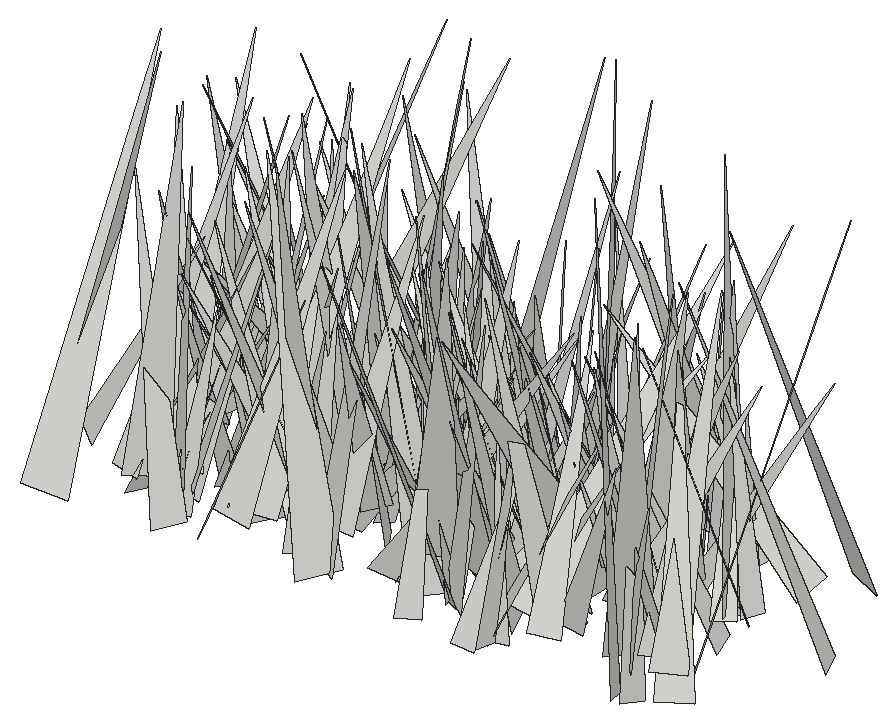
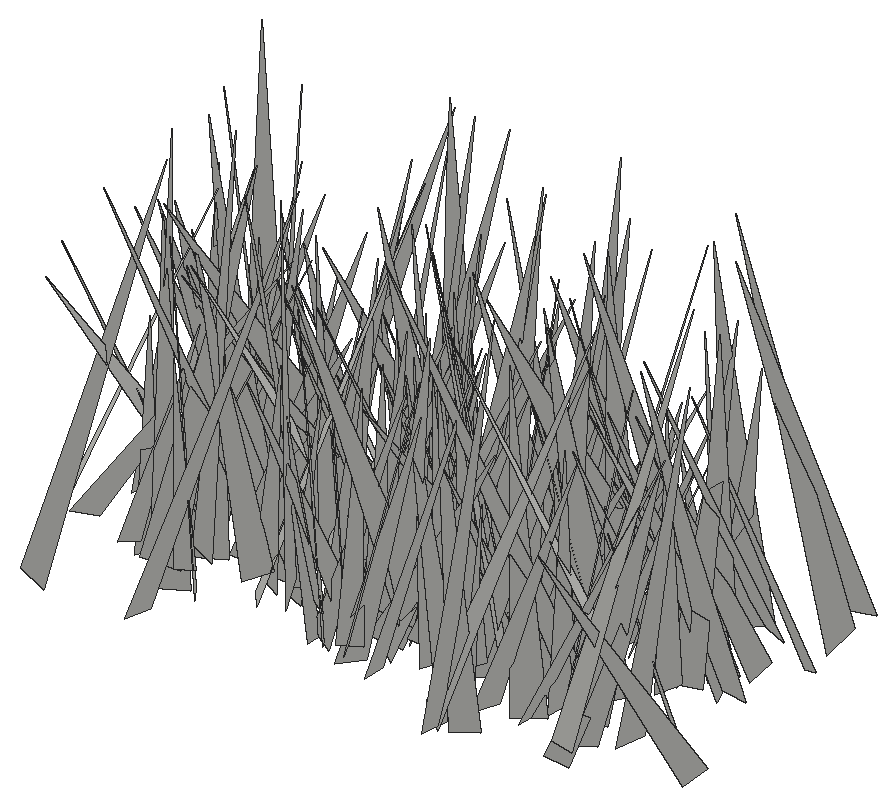
# SketchUp Ruby script. Lengths in inches.
U = 1.inch
M = Sketchup.active_model
def pt(a) = Geom::Point3d.new(a.map { |v| v * U })
def face(e, loops, mat)
  f = e.add_face(loops[0].map { |a| pt(a) })
  loops[1..].each { |l| e.add_face(l.map { |a| pt(a) }).erase! }
  f.material = f.back_material = mat if mat
  f
end
# faces: each face lists its corners as indices into pts; further lists are holes
def faces(e, pts, list, mat = nil) = list.each { |f| face(e, (f[0].is_a?(Array) ? f : [f]).map { |l| l.map { |i| pts[i] } }, mat) }
# xy, xz, yz: faces in a plane at the given z, y or x. An outline is a flat list of corners, or four numbers for a rectangle; further outlines are holes
def ring(l) = l.size == 4 ? [[l[0], l[1]], [l[2], l[1]], [l[2], l[3]], [l[0], l[3]]] : l.each_slice(2).to_a
def flat(e, list, mat, &to3) = list.each { |f| face(e, (f[0].is_a?(Array) ? f : [f]).map { |l| ring(l).map { |u, v| to3.(u, v) } }, mat) }
def xy(e, z, list, mat = nil) = flat(e, list, mat) { |x, y| [x, y, z] }
def xz(e, y, list, mat = nil) = flat(e, list, mat) { |x, z| [x, y, z] }
def yz(e, x, list, mat = nil) = flat(e, list, mat) { |y, z| [x, y, z] }
def lines(e, pts, list) = list.each { |a, b| e.add_line(pt(pts[a]), pt(pts[b])) }
# prism: a flat outline (further loops are holes) pulled along v
def prism(e, loops, v, mat = nil)
  f = face(e, loops, mat); d = Geom::Vector3d.new(v.map { |x| x * U })
  f.pushpull(f.normal.samedirection?(d) ? d.length : -d.length)
end
def box(e, o, s, mat = nil) = prism(e, [[o, [o[0] + s[0], o[1], o[2]], [o[0] + s[0], o[1] + s[1], o[2]], [o[0], o[1] + s[1], o[2]]]], [0, 0, s[2]], mat)
def at(x, y, z, deg = 0) = Geom::Transformation.translation(pt([x, y, z])) * Geom::Transformation.rotation(ORIGIN, Z_AXIS, deg.degrees)
def axes(o, x, y, z) = Geom::Transformation.new([*x, 0, *y, 0, *z, 0, *pt(o).to_a, 1])
def part(name) = M.definitions.add(name)
# library, detail: a bought-in or finely detailed component or shape, given as its bounding box
def library(name, o, s) = part(name).tap { |d| box(d.entities, o, s) }
def detail(e, o, s) = box(e.add_group.entities, o, s)
def put(e, d, t, mat = nil) = e.add_instance(d, t).tap { |i| i.material = mat if mat }
def group(e, t, mat = nil) = e.add_group.tap { |g| g.transformation = t; g.material = mat if mat }.entities
root = M.entities
c1 = part("fur_instance\#9")
p = [[0.8125,0,1.79],[0.67,-0.02,1.48],[0,-0.11,0],[0,0.11,0]]
faces(c1.entities,p,[[0,1,2,3]])
put(root,c1,axes([89.15,61.55,-27.1],[-1.14842,8.02715,0.79991],[8.02073,1.22255,-0.75306],[0.86188,-0.68125,8.07384]))
put(root,c1,axes([101.82,65.9,-27.1],[5.04429,-5.44094,0.7168],[-5.46997,-5.06343,0.05905],[-0.44381,0.56596,7.41924]))
put(root,c1,axes([88.16,63.39,-27.1],[7.83085,1.1219,1.78667],[1.00117,-8.02181,0.64907],[-1.85702,0.40616,7.88414]))
put(root,c1,axes([108.1,65.12,-27.1],[1.41621,-4.16021,0.5332],[-4.01988,-1.18575,1.42542],[1.19673,0.94019,4.15706]))
put(root,c1,axes([105.11,66.26,-28.22],[-5.97447,-2.65496,2.2585],[-2.10106,6.3191,1.8704],[2.78122,-0.92951,6.26456]))
put(root,c1,axes([96.97,65.74,-27.1],[-0.69172,-7.26259,1.83893],[-7.46362,0.82804,0.46276],[0.64909,1.78171,7.28077]))
put(root,c1,axes([109.4375,66.59,-28.22],[5.80631,-5.6916,0.53269],[-5.68589,-5.82856,-0.29992],[-0.59055,0.15799,8.12513]))
put(root,c1,axes([104.92,63.54,-28.22],[-0.85161,3.55792,0.87868],[3.50079,1.05663,-0.88551],[1.08413,-0.61714,3.54963]))
put(root,c1,axes([107.41,65.17,-27.1],[-5.83631,0.9789,1.84731],[1.28037,6.00401,0.86359],[1.65271,-1.19453,5.85448]))
put(root,c1,axes([105.4375,64.125,-28.22],[3.9323,-0.29865,1.47953],[-0.48436,-4.16008,0.44758],[-1.42954,0.58799,3.91814]))
put(root,c1,axes([98.31,64.36,-28.22],[5.34271,-3.44394,4.19103],[-3.85612,-6.54857,-0.46545],[-3.8152,1.796,6.33945]))
put(root,c1,axes([112.05,62.54,-27.1],[-7.32928,-2.99407,2.48715],[-3.76161,6.81126,-2.88543],[1.00033,3.67572,7.37273]))
put(root,c1,axes([102.34,63.93,-28.22],[-2.63101,2.88231,1.12737],[2.88894,2.81797,-0.46255],[1.11028,-0.50218,3.87505]))
put(root,c1,axes([91.07,64.46,-27.1],[4.75602,-4.66812,2.75377],[-5.20371,-4.95731,0.58378],[-1.51526,2.37234,6.63855]))
put(root,c1,axes([92.46,63.86,-28.22],[-5.69821,2.17721,0.97614],[2.15034,5.78116,-0.34192],[1.034,-0.02439,6.0904]))
put(root,c1,axes([103.32,67.53,-28.22],[-1.56855,-7.63886,0.47282],[-7.63369,1.59619,0.46371],[0.55001,0.36889,7.78444]))
put(root,c1,axes([102.75,67.41,-28.22],[-1.24529,-7.71146,0.7872],[-7.61167,1.36728,1.35282],[1.46589,0.54863,7.69333]))
put(root,c1,axes([105.64,64.5,-28.22],[-0.42673,3.51272,1.26133],[3.73148,0.37463,0.21911],[-0.0791,-1.27778,3.53176]))
put(root,c1,axes([95.66,67.33,-28.22],[-5.87667,-3.9224,1.1719],[-3.54254,5.90008,1.98324],[2.05159,-1.04767,6.78139]))
put(root,c1,axes([106.1,69.67,-28.22],[6.48177,-5.01878,0.45242],[-4.24735,-5.8379,-3.90962],[-2.71162,-2.85253,7.2053]))
put(root,c1,axes([92.17,64.72,-28.22],[1.50954,-3.07856,1.78204],[-3.55315,-1.39659,0.59714],[-0.16832,1.87187,3.37633]))
put(root,c1,axes([111.02,64.51,-27.1],[4.54729,4.68314,2.12923],[4.88324,-4.82336,0.17985],[-1.61844,-1.39522,6.52513]))
put(root,c1,axes([105.03,64.76,-28.22],[4.26257,2.91433,0.00484],[2.86478,-4.18851,-0.95515],[0.53516,-0.79116,5.0745]))
put(root,c1,axes([102.89,65.54,-28.22],[-4.07281,-4.5818,0.7427],[-4.55178,3.7491,-1.83244],[-0.90871,1.75604,5.85003]))
put(root,c1,axes([112.17,65.62,-28.22],[-2.82559,-5.19892,1.36333],[-5.31081,2.46391,-1.61114],[-0.82624,1.9421,5.69358]))
put(root,c1,axes([92.14,64.79,-27.1],[3.06348,4.37723,2.06786],[4.6001,-3.39453,0.37061],[-1.50841,-1.46222,5.32989]))
put(root,c1,axes([102.83,65.68,-28.22],[-2.2184,-4.85625,2.50772],[-5.03427,2.86928,1.10295],[2.1279,1.72546,5.22379]))
put(root,c1,axes([97.12,66.88,-27.1],[-5.96376,-1.66281,1.60864],[-1.32131,6.09893,1.40577],[1.89916,-0.97833,6.02952]))
put(root,c1,axes([93.52,64.26,-28.22],[4.67763,2.46387,0.32375],[2.42875,-4.67875,0.51598],[-0.52599,0.30722,5.26162]))
put(root,c1,axes([98.24,67.43,-27.1],[3.42227,-3.49613,0.30492],[-3.40506,-3.41104,-0.89344],[-0.84941,-0.41195,4.81005]))
put(root,c1,axes([94.98,63.97,-27.1],[0.10942,6.44965,1.02032],[6.44115,0.06102,-1.07648],[1.07264,-1.02435,6.36012]))
put(root,c1,axes([87.73,65.51,-27.1],[2.82226,4.09729,0.68802],[3.94816,-2.38599,-1.98631],[1.29353,-1.65697,4.56152]))
put(root,c1,axes([97.99,64.9,-28.22],[3.51282,6.48869,2.15536],[6.79895,-3.57131,-0.32959],[-0.72316,-2.057,7.37118]))
put(root,c1,axes([103.6875,68.1875,-28.22],[0.91658,-6.09487,0.23316],[-5.96683,-0.94489,-1.24341],[-1.26442,0.04079,6.03668]))
put(root,c1,axes([107.76,64.21,-27.1],[-1.60174,4.9541,0.61833],[4.97114,1.64265,-0.28364],[0.46172,-0.4996,5.19887]))
put(root,c1,axes([92.63,64.84,-27.1],[3.7464,3.46532,0.67043],[3.46985,-3.79505,0.22613],[-0.64655,-0.28736,5.09832]))
put(root,c1,axes([94.75,66.3125,-28.22],[-5.61419,2.77509,3.47904],[3.15086,6.4338,-0.04739],[3.14276,-1.49299,6.26243]))
put(root,c1,axes([96.64,67.13,-28.22],[-3.76268,-4.24685,0.11424],[-4.17448,3.66755,-1.15295],[-0.78896,0.84846,5.55555]))
put(root,c1,axes([90.15,65.0625,-28.22],[5.14686,-0.10254,0.48257],[-0.21946,-5.00543,1.27711],[-0.44184,1.29176,4.98695]))
put(root,c1,axes([91.81,65.32,-27.1],[-3.36286,5.21282,1.50099],[5.38655,3.41774,0.19865],[0.64152,-1.37145,6.20023]))
put(root,c1,axes([92.19,67.5,-28.22],[-0.08561,-4.51883,0.61864],[-4.55746,0.06047,-0.18896],[-0.17898,0.62161,4.51569]))
put(root,c1,axes([102.125,65.86,-28.22],[-4.38445,3.57185,1.79964],[3.76738,4.58485,0.07863],[1.34299,-1.20052,5.65467]))
put(root,c1,axes([111.46,64.16,-28.22],[-6.16922,0.32467,1.04524],[-0.06119,5.87189,-2.18505],[1.09279,2.16166,5.77844]))
put(root,c1,axes([102.52,66,-28.22],[-6.07164,-2.28107,2.04855],[-2.55827,6.27412,-0.5961],[1.68971,1.3026,6.45854]))
put(root,c1,axes([105.42,67.24,-27.1],[3.7363,2.07589,0.22504],[1.88074,-3.14536,-2.2112],[0.90706,-2.02911,3.65784]))
put(root,c1,axes([100.69,68.03,-28.22],[-1.13114,-4.608,0.05517],[-4.59723,1.12439,-0.34274],[-0.31976,0.13515,4.73241]))
put(root,c1,axes([100.07,66.25,-28.22],[4.34126,2.62004,0.01209],[2.52851,-4.18338,-1.34808],[0.68659,-1.1602,4.88813]))
put(root,c1,axes([100.05,65.7,-28.22],[4.70359,-4.43483,0.77561],[-4.1988,-3.91632,3.07011],[1.62462,2.71804,5.6891]))
put(root,c1,axes([112.55,65,-28.22],[-3.10471,5.12305,0.88051],[5.18598,3.12286,0.11631],[0.35573,-0.81381,5.98927]))
put(root,c1,axes([90.27,68.8125,-27.1],[0.60186,-6.09784,0.10298],[-6.0697,-0.58883,0.60707],[0.59415,0.16161,6.09732]))
put(root,c1,axes([93.92,68.03,-27.1],[-4.12735,0.23871,1.0618],[0.66209,3.85593,1.70672],[0.86374,-1.81501,3.76552]))
put(root,c1,axes([98.74,67.43,-28.22],[-4.89402,-3.33819,1.83703],[-3.30827,5.20635,0.64726],[1.89038,0.46913,5.88863]))
put(root,c1,axes([109.83,68.41,-28.22],[-3.94207,-4.94022,1.13908],[-4.81769,4.09962,1.10733],[1.57897,0.1748,6.2225]))
put(root,c1,axes([98.04,65.56,-27.1],[-0.68675,5.73435,1.62653],[5.78722,1.03346,-1.2],[1.42703,-1.4315,5.64928]))
put(root,c1,axes([95.05,66.89,-28.22],[3.78435,-1.32179,0.68035],[-1.35222,-3.83372,0.07338],[-0.61764,0.29457,4.00787]))
put(root,c1,axes([102.03,66.07,-28.22],[-1.02594,6.32348,2.52203],[6.58274,1.57191,-1.26344],[1.73626,-2.22313,6.28034]))
put(root,c1,axes([100.82,67.67,-28.22],[1.24719,-3.91493,0.4967],[-3.8954,-1.13791,0.81231],[0.63182,0.71228,4.02769]))
put(root,c1,axes([102.06,67.64,-28.22],[-1.33091,-4.34516,1.37723],[-4.35803,1.6335,0.94222],[1.33595,0.99989,4.44566]))
put(root,c1,axes([108.55,68.06,-27.1],[4.51587,-1.82573,1.61231],[-1.49442,-4.75873,-1.20297],[-1.92343,-0.58918,4.72009]))
put(root,c1,axes([95.08,66.96,-28.22],[0.69074,-4.72184,2.34998],[-4.89788,-1.45354,-1.48096],[-1.95676,1.97148,4.53648]))
put(root,c1,axes([90.75,65.92,-28.22],[4.0967,-0.1052,0.02727],[-0.10864,-3.93802,1.12914],[0.00278,1.12946,3.93942]))
put(root,c1,axes([90.3125,64.27,-27.1],[2.22729,6.28936,0.04999],[6.2767,-2.22605,0.40869],[-0.40191,0.08939,6.65956]))
put(root,c1,axes([100.12,67.4375,-27.1],[4.02018,4.80904,4.066],[5.52928,-5.00439,0.45193],[-3.01434,-2.76593,6.25176]))
put(root,c1,axes([96.04,66.42,-28.22],[-2.33068,3.85921,0.35584],[3.66264,2.05758,1.6744],[-1.26695,-1.15111,4.18592]))
put(root,c1,axes([91.125,66.02,-28.22],[0.24663,7.62872,2.41582],[7.70784,0.42293,-2.12242],[2.15005,-2.39126,7.33168]))
put(root,c1,axes([106.17,68.05,-28.22],[-2.38494,-6.16406,1.52656],[-6.35023,2.30898,-0.59758],[-0.0234,1.63919,6.58229]))
put(root,c1,axes([94.38,66.36,-28.22],[-3.84784,-1.19504,0.32807],[-1.23606,3.62421,-1.29571],[-0.08892,1.33363,3.81512]))
put(root,c1,axes([94.29,65.36,-27.1],[4.06792,5.19434,1.22411],[5.14399,-4.22635,0.83955],[-1.42088,-0.42943,6.54403]))
put(root,c1,axes([100.61,66.89,-27.1],[0.55965,-6.1533,3.26603],[-6.71098,-1.35523,-1.40332],[-1.86889,3.02383,6.01722]))
put(root,c1,axes([108.04,68.29,-28.22],[-3.36385,-0.86607,1.07357],[-0.51946,3.41676,1.12873],[1.27781,-0.89095,3.28504]))
put(root,c1,axes([104.87,67.96,-28.22],[-3.34237,-3.67886,0.49489],[-3.71061,3.29315,-0.58039],[-0.10119,0.75599,4.93646]))
put(root,c1,axes([93.67,68.76,-28.22],[-3.17916,-2.57933,0.00353],[-2.53731,3.12837,0.73174],[0.46373,-0.56605,4.02798]))
put(root,c1,axes([106.79,67.59,-28.22],[-3.3946,-3.12525,1.18102],[-3.29173,3.41661,-0.4203],[0.5714,1.11577,4.59499]))
put(root,c1,axes([112.45,64.78,-27.1],[-5.42402,3.35952,0.54018],[3.08821,5.28712,-1.87283],[1.42868,1.32596,6.09909]))
put(root,c1,axes([106.79,69.17,-27.1],[1.2889,-4.23263,0.01136],[-4.22076,-1.28617,-0.32791],[-0.31699,-0.08469,4.41236]))
put(root,c1,axes([111.32,65.36,-27.1],[-4.3486,2.21974,0.80785],[1.83051,4.23636,-1.78683],[1.49303,1.27131,4.54366]))
put(root,c1,axes([107.68,69.69,-28.22],[2.24091,-5.47361,0.67385],[-5.23088,-2.33999,-1.61199],[-1.7471,-0.01469,5.69066]))
put(root,c1,axes([99.96,67.06,-28.22],[4.49912,0.07902,0.02983],[0.07502,-4.46879,0.52292],[-0.03881,0.52233,4.46932]))
put(root,c1,axes([103.45,67.43,-27.1],[-3.94466,-0.14605,1.57067],[-0.23954,4.23653,-0.20765],[1.55915,0.28136,3.94189]))
put(root,c1,axes([111.99,69.36,-27.1],[-3.65311,-4.50937,0.62916],[-4.48426,3.70309,0.50402],[0.78847,0.16789,5.78149]))
put(root,c1,axes([99.7,68.51,-28.22],[1.8485,-3.49978,1.33816],[-3.45042,-2.17169,-0.91344],[-1.46071,0.70098,3.8511]))
put(root,c1,axes([108.77,67.17,-27.1],[0.87918,5.14411,1.43079],[4.85097,-0.16366,-2.39235],[2.23095,-1.67133,4.63805]))
put(root,c1,axes([107.97,68.7,-28.22],[2.2039,-6.87435,1.74953],[-7.02125,-1.85328,1.56272],[1.00974,2.1174,7.04782]))
put(root,c1,axes([108.61,67.74,-27.1],[-0.27177,-3.75184,1.87256],[-3.70908,-0.66019,-1.86105],[-1.95589,1.77327,3.26904]))
put(root,c1,axes([105.58,67.75,-28.22],[-0.77186,4.35622,1.72795],[4.2436,-0.09339,2.13104],[-1.98854,-1.8902,3.87699]))
put(root,c1,axes([111.4,68.96,-28.22],[-5.35424,-1.86738,0.02315],[-1.86377,5.3475,0.29345],[0.11847,-0.26947,5.66294]))
put(root,c1,axes([96.78,70.72,-28.22],[7.37439,-3.31849,1.28024],[-2.90244,-7.31769,-2.24953],[-2.05603,-1.57231,7.76747]))
put(root,c1,axes([104.125,65.94,-28.22],[0.90469,6.24799,0.05202],[5.52251,-0.775,-2.9597],[2.92267,-0.46962,5.57638]))
put(root,c1,axes([96.52,68.87,-27.1],[-6.02473,-0.71032,1.74625],[-0.51818,6.24626,0.75302],[1.81257,-0.57532,6.01954]))
put(root,c1,axes([97.01,65.1875,-28.22],[-7.34828,2.49323,1.09592],[2.03506,7.1224,-2.5582],[1.80991,2.11416,7.32591]))
put(root,c1,axes([101.71,67.9,-27.1],[-4.44101,1.77663,0.66677],[1.83519,4.45274,0.3588],[0.48276,-0.58331,4.76973]))
put(root,c1,axes([106.6,65.01,-27.1],[-2.65177,6.66161,0.65253],[5.97681,2.67255,-2.995],[3.01341,0.56142,6.51452]))
put(root,c1,axes([100.72,67.9,-27.1],[2.95433,4.07724,0.35212],[3.82019,-2.59183,-2.04072],[1.46767,-1.46099,4.60298]))
put(root,c1,axes([93.55,68.56,-27.1],[4.21997,-0.6182,0.41958],[-0.60999,-4.24047,-0.11271],[-0.43142,-0.05127,4.26352]))
put(root,c1,axes([104.69,69.3,-27.1],[5.27182,0.13194,1.25121],[0.40362,-5.28245,-1.14356],[-1.19165,-1.2055,5.14798]))
put(root,c1,axes([99.09,69.38,-28.22],[2.10827,-4.41232,0.88185],[-4.4927,-2.11805,0.1432],[-0.24874,0.85808,4.88803]))
put(root,c1,axes([102.77,68.04,-28.22],[1.63148,3.88333,0.8996],[3.80186,-1.22375,-1.61232],[1.19808,-1.40479,3.89132]))
put(root,c1,axes([108.88,70.32,-28.22],[1.92624,-6.27783,0.49509],[-6.26935,-1.863,0.76884],[0.59288,0.69623,6.52153]))
put(root,c1,axes([95.3,64.65,-27.1],[-5.76444,5.45156,1.05869],[4.71185,5.60881,-3.22628],[2.93919,1.70025,7.24841]))
put(root,c1,axes([102.25,68.26,-27.1],[-2.34318,3.21724,1.23905],[3.43189,2.31946,0.46753],[0.3286,-1.2829,3.95253]))
put(root,c1,axes([102.86,71.12,-28.22],[5.45875,-2.61976,0.1584],[-2.41646,-5.15945,-2.05595],[-1.02417,-1.78972,5.6951]))
put(root,c1,axes([91.68,65.67,-27.1],[4.88269,3.53574,0.69101],[3.04894,-4.67553,2.3797],[-1.91908,1.56767,5.53887]))
put(root,c1,axes([105.96,71.46,-28.22],[-5.79035,-4.99721,0.36352],[-4.82955,5.71454,1.62848],[1.33407,-1.00217,7.47317]))
put(root,c1,axes([94.84,70.11,-28.22],[2.46891,-7.20313,1.70316],[-7.36136,-2.57683,-0.22704],[-0.77207,1.53499,7.61111]))
put(root,c1,axes([94.51,67.79,-28.22],[3.62084,3.81527,1.03017],[3.87963,-3.69771,0.05854],[-0.75237,-0.70613,5.25959]))
put(root,c1,axes([103.54,68.75,-27.1],[-3.16425,3.77948,0.90882],[3.82647,2.82214,1.58634],[-0.68447,-1.69527,4.66695]))
put(root,c1,axes([107.28,68.91,-28.22],[3.73995,-4.97965,1.07609],[-4.97131,-3.27521,2.12161],[1.114,2.10195,5.85517]))
put(root,c1,axes([90.46,66.51,-28.22],[5.94248,2.0649,1.47313],[1.51819,-5.90154,2.14801],[-2.032,1.62942,5.91295]))
put(root,c1,axes([92.16,67.11,-28.22],[4.99403,0.89918,1.35491],[0.3935,-4.91429,1.81096],[-1.5778,1.62046,4.74018]))
put(root,c1,axes([97.02,67.5,-28.22],[4.61387,-2.10989,0.31356],[-1.93342,-3.82099,2.73855],[0.90102,2.60502,4.2708]))
put(root,c1,axes([97.74,68.44,-28.22],[3.36091,-1.13304,0.9234],[-1.35023,-3.29337,0.87337],[-0.55977,1.1411,3.43755]))
put(root,c1,axes([90.54,69.36,-27.1],[4.66089,-0.94094,1.87831],[-0.93791,-5.02216,-0.1885],[-1.87983,0.17273,4.75118]))
put(root,c1,axes([99.8,67.64,-27.1],[2.15657,3.40289,0.33157],[3.29952,-2.17412,0.8525],[-0.89598,0.18416,3.93747]))
put(root,c1,axes([90.1875,66.76,-28.22],[0.44326,7.59594,0.73525],[7.62112,-0.4789,0.35297],[-0.39679,-0.71255,7.60067]))
put(root,c1,axes([93.79,69,-27.1],[-4.37438,2.14658,0.79892],[2.22863,4.38643,0.41683],[0.52851,-0.72986,4.85482]))
put(root,c1,axes([106.63,66.29,-27.1],[4.76717,4.34009,0.09976],[4.0907,-4.54047,2.05487],[-1.45344,1.45601,6.11063]))
put(root,c1,axes([104.82,69.5,-27.1],[-3.19994,-2.12817,0.10035],[-2.08753,3.09569,-0.91527],[-0.42587,0.81635,3.73243]))
put(root,c1,axes([96.49,70.26,-28.22],[-2.52034,-4.28654,0.32351],[-4.12689,2.30776,-1.57296],[-1.20326,1.06349,4.71724]))
put(root,c1,axes([114.95,70.09,-28.22],[-6.30191,-3.29477,0.26908],[-3.30318,6.25333,-0.79169],[-0.13009,0.82599,7.06702]))
put(root,c1,axes([100.36,70.35,-28.22],[-4.19066,-2.50752,1.09961],[-2.47633,4.32875,0.43379],[1.16817,0.18082,4.86427]))
put(root,c1,axes([104.24,66.26,-28.22],[3.62911,6.60842,0.2466],[6.35712,-3.56375,1.94657],[-1.82181,0.72867,7.28371]))
put(root,c1,axes([94.13,69.76,-27.1],[2.50338,-2.82714,1.30611],[-3.05988,-2.54469,0.35667],[-0.57944,1.22368,3.75931]))
put(root,c1,axes([93.97,70.69,-27.1],[-1.02707,-3.52995,0.46815],[-3.49734,0.90838,-0.82343],[-0.66956,0.66999,3.58293]))
put(root,c1,axes([101.92,70.31,-27.1],[0.28904,-4.61969,1.68996],[-4.89331,-0.44312,-0.3744],[-0.50298,1.65624,4.61355]))
put(root,c1,axes([111.68,68.61,-27.1],[-2.57238,2.98987,0.10946],[2.97729,2.57237,-0.29516],[0.29502,0.10983,3.93311]))
put(root,c1,axes([92.85,69.58,-28.22],[5.12672,-4.5376,2.59386],[-5.0883,-5.16347,1.02416],[-1.19461,2.5199,6.76936]))
put(root,c1,axes([98.65,72.02,-27.1],[1.56687,-4.2825,0.24372],[-4.04586,-1.5617,-1.43053],[-1.42486,-0.27491,4.32996]))
put(root,c1,axes([100.66,71.47,-28.22],[-3.68425,-5.36529,0.32526],[-5.32374,3.58793,-1.11818],[-0.74155,0.8979,6.41168]))
put(root,c1,axes([112.21,69.49,-27.1],[-4.36363,0.98227,0.81119],[0.91976,4.432,-0.41906],[0.88144,0.23814,4.45315]))
put(root,c1,axes([97.375,68.96,-27.1],[5.30824,4.83924,1.79848],[4.88732,-5.54151,0.48577],[-1.6634,-0.83881,7.16657]))
put(root,c1,axes([97.09,71.49,-27.1],[0.61294,-5.47928,1.38132],[-5.30961,-1.0339,-1.7451],[-1.93355,1.10218,5.22999]))
put(root,c1,axes([104.96,70.75,-28.22],[-1.22069,-3.41408,1.05948],[-3.55821,1.26785,-0.01408],[0.34288,1.00256,3.62571]))
put(root,c1,axes([101.37,70.98,-28.22],[-3.20699,2.34244,2.63387],[2.95903,3.72406,0.29089],[1.91533,-1.83124,3.96071]))
put(root,c1,axes([112.61,72.05,-27.1],[-5.96221,1.49508,0.02596],[1.36332,5.39133,2.61894],[-0.61423,-2.54602,5.56097]))
put(root,c1,axes([105.02,70.68,-28.22],[-0.92871,-3.83483,1.6083],[-4.04735,1.2119,0.55253],[0.95473,1.40727,3.90681]))
put(root,c1,axes([109.48,70.04,-27.1],[3.29682,4.04593,0.27696],[3.82738,-2.98619,-1.93627],[1.34069,-1.42422,4.84659]))
put(root,c1,axes([111.5,69.35,-27.1],[-7.33304,-1.55705,2.53328],[-2.07568,7.50758,-1.39398],[2.1292,1.95633,7.36578]))
put(root,c1,axes([91.66,73.78,-28.22],[4.40481,-2.70951,0.82389],[-1.71706,-3.76665,-3.20728],[-2.2521,-2.42766,4.05674]))
put(root,c1,axes([89.78,69.91,-28.22],[2.28219,3.09258,0.57784],[3.14608,-2.24088,-0.43237],[0.01087,-0.72161,3.81909]))
put(root,c1,axes([90.58,71.28,-28.22],[-6.33484,-0.15602,2.15214],[0.09289,6.64883,0.75543],[2.15578,-0.74496,6.29157]))
put(root,c1,axes([98.47,70.94,-28.22],[0.02782,-4.7345,1.86898],[-5.06027,0.17616,0.52158],[0.54982,1.86087,4.70577]))
put(root,c1,axes([107.93,71.81,-27.1],[-3.27673,-6.38483,2.25273],[-6.55108,3.62196,0.73666],[1.71005,1.64109,7.13865]))
put(root,c1,axes([110.67,71.22,-28.22],[3.6892,-1.49713,1.29137],[-1.47127,-3.90506,-0.32413],[-1.32076,0.16824,3.96818]))
put(root,c1,axes([96.43,72.11,-27.1],[6.1777,-0.38175,1.16241],[-0.13775,-6.16226,-1.29169],[-1.21571,-1.24165,6.0532]))
put(root,c1,axes([108.61,73.13,-27.1],[1.25653,-6.81976,0.6894],[-6.81087,-1.32116,-0.65555],[-0.77223,0.55558,6.90349]))
put(root,c1,axes([92.72,71.94,-27.1],[-4.52954,-3.25843,1.35312],[-3.24257,4.71245,0.49358],[1.39071,0.3748,5.55792]))
put(root,c1,axes([90.9,74.46,-27.1],[-3.5223,-6.70382,0.02091],[-6.50166,3.42181,1.83516],[1.63401,-0.83562,7.34711]))
put(root,c1,axes([105.59,71.84,-27.1],[5.75538,-1.33671,0.29214],[-1.31847,-5.75568,-0.36093],[-0.36579,-0.28603,5.89753]))
put(root,c1,axes([96.39,69.46,-27.1],[-0.08905,4.06249,0.07241],[4.03019,0.09752,-0.5148],[0.51634,-0.06053,4.03072]))
put(root,c1,axes([94.14,72.1,-28.22],[2.19919,-5.46865,1.19281],[-5.58851,-2.07385,0.79564],[0.31218,1.39943,5.84033]))
put(root,c1,axes([94.11,72.11,-28.22],[-5.87087,-0.65311,0.1721],[-0.62527,5.82501,0.77566],[0.25536,-0.75237,5.85594]))
put(root,c1,axes([106.1,69.97,-28.22],[3.12045,6.97557,0.92804],[6.87353,-2.80376,-2.03727],[1.5081,-1.6545,7.36514]))
put(root,c1,axes([91.6,72.41,-28.22],[-4.18916,1.41328,1.44955],[1.84035,4.04661,1.3732],[0.84361,-1.80976,4.20247]))
put(root,c1,axes([96.22,70.85,-27.1],[6.38411,4.40631,2.11358],[4.61615,-6.57865,-0.22824],[-1.60436,-1.39477,7.75373]))
put(root,c1,axes([112.03,66.56,-28.22],[5.94606,5.36025,0.59468],[4.2161,-5.17199,4.4628],[-3.36309,2.9933,6.64615]))
put(root,c1,axes([93.71,70.93,-28.22],[-5.13165,1.21269,1.54361],[1.09048,5.35359,-0.58061],[1.63224,0.23592,5.24093]))
put(root,c1,axes([108.56,72.69,-28.22],[2.3512,-5.85332,1.44977],[-6.03015,-2.28819,0.5412],[-0.02311,1.54732,6.28463]))
put(root,c1,axes([97.61,73.0625,-27.1],[4.97524,0.71585,1.07536],[1.04452,-4.74693,-1.67259],[-0.76015,-1.83742,4.74004]))
put(root,c1,axes([102.58,72.1875,-28.22],[4.61711,2.95667,1.94744],[3.35791,-4.67134,-0.86895],[-1.12198,-1.8135,5.41336]))
put(root,c1,axes([110.31,72.61,-27.1],[-3.89042,0.9571,1.21715],[1.27935,3.84105,1.06884],[0.87221,-1.36496,3.86121]))
put(root,c1,axes([92.53,71.11,-28.22],[-3.78677,4.88862,0.77178],[4.90876,3.58599,1.37062],[-0.63111,-1.44081,6.0299]))
put(root,c1,axes([100.92,71.07,-28.22],[-3.06534,4.86368,0.18481],[4.51167,2.75744,2.26433],[-1.82603,-1.35165,5.28436]))
put(root,c1,axes([102.82,72.39,-28.22],[4.30698,0.82715,0.77594],[0.97071,-4.26434,-0.84231],[-0.5865,-0.98365,4.30404]))
put(root,c1,axes([102.69,72.2,-28.22],[-2.4507,-4.58404,1.24543],[-4.71435,2.17524,-1.27033],[-0.58261,1.68089,5.0404]))
put(root,c1,axes([107.74,72.39,-28.22],[4.89735,3.35239,2.18214],[3.80193,-4.97328,-0.89225],[-1.24321,-2.00306,5.86741]))
put(root,c1,axes([93.42,70.66,-27.1],[2.59444,7.48207,1.23534],[7.31718,-2.12705,-2.48457],[1.99156,-1.93206,7.51927]))
put(root,c1,axes([106.48,70.35,-28.22],[1.00631,5.78428,1.17144],[5.41169,-1.37849,2.15781],[-2.35451,-0.6962,5.46025]))
put(root,c1,axes([100.42,73.54,-27.1],[1.67975,-3.93598,0.16611],[-3.93538,-1.66827,0.26597],[0.17974,0.25696,4.27115]))
put(root,c1,axes([100.32,71.2,-27.1],[-1.21025,6.4146,1.42422],[6.45546,0.89059,1.47445],[-1.22575,-1.64315,6.35907]))
put(root,c1,axes([91.96,69.84,-27.1],[5.80303,5.01805,0.27093],[4.96083,-5.78629,0.91567],[-0.80277,0.51711,7.61693]))
put(root,c1,axes([96.68,73.92,-28.22],[-4.99858,-6.00178,0.67378],[-6.03784,4.94565,-0.739],[-0.1407,0.9901,7.77567]))
put(root,c1,axes([108.35,74.61,-28.22],[-7.7703,-1.5883,1.42664],[-1.2052,7.70803,2.01725],[1.76224,-1.7318,7.67014]))
put(root,c1,axes([95.66,72.44,-28.22],[-5.48132,1.03762,0.48302],[1.07413,5.47965,0.41785],[0.39525,-0.50168,5.563]))
put(root,c1,axes([107.73,72.97,-27.1],[0.85171,-3.4207,0.8533],[-3.50883,-0.73716,0.54719],[0.34265,0.95401,3.48241]))
put(root,c1,axes([96.66,73.01,-28.22],[5.5976,-0.64404,1.05715],[-0.59203,-5.69245,-0.3332],[-1.08713,-0.21617,5.62467]))
put(root,c1,axes([101.58,72.38,-27.1],[3.14318,2.78213,1.66083],[2.96777,-3.40061,0.07991],[-1.30037,-1.03624,4.19683]))
put(root,c1,axes([87.49,71.78,-28.22],[3.92135,-2.35365,0.03406],[-2.05535,-3.39138,2.27856],[1.14733,1.96892,3.96545]))
put(root,c1,axes([103.09,71.99,-27.1],[4.37398,5.97616,2.1686],[6.29129,-4.44766,-0.43255],[-0.91492,-2.01317,7.39318]))
put(root,c1,axes([102.34,71.41,-27.1],[4.56042,0.58445,0.815],[0.35248,-4.48653,1.24501],[-0.93891,1.15443,4.42595]))
put(root,c1,axes([95.2,74.11,-28.22],[0.81031,-5.69395,0.84212],[-5.55553,-0.55126,1.61834],[1.50543,1.03047,5.51893]))
put(root,c1,axes([112.48,74.95,-28.22],[-3.23676,-6.95107,0.75182],[-6.9834,3.25434,0.02332],[0.33861,0.67166,7.66769]))
put(root,c1,axes([95.43,73.79,-28.22],[-0.85908,-3.57953,0.71794],[-3.54097,0.99653,0.73143],[0.88884,0.51028,3.60778]))
put(root,c1,axes([100.98,72.78,-28.22],[-4.79619,2.23097,0.90337],[2.34699,4.78153,0.65218],[0.53379,-0.97799,5.24932]))
put(root,c1,axes([100.34,73.8,-27.1],[-4.23671,-2.59002,0.97553],[-2.55905,4.34534,0.42292],[1.0541,0.13924,4.94763]))
put(root,c1,axes([104.03,72.08,-27.1],[-6.60957,-3.13791,3.29203],[-3.79035,7.01015,-0.92809],[2.51341,2.31982,7.25752]))
put(root,c1,axes([98.69,74.47,-27.1],[-5.81258,-1.56867,1.18702],[-1.32265,5.85738,1.26392],[1.45614,-0.94136,5.88637]))
put(root,c1,axes([96.14,74.49,-28.22],[6.50516,0.09741,3.11354],[0.81371,-7.01185,-1.48071],[-3.00691,-1.68675,6.33514]))
put(root,c1,axes([100.27,70.46,-27.1],[7.12046,1.58475,2.39098],[0.70942,-7.17277,2.64146],[-2.77938,2.22916,6.79964]))
